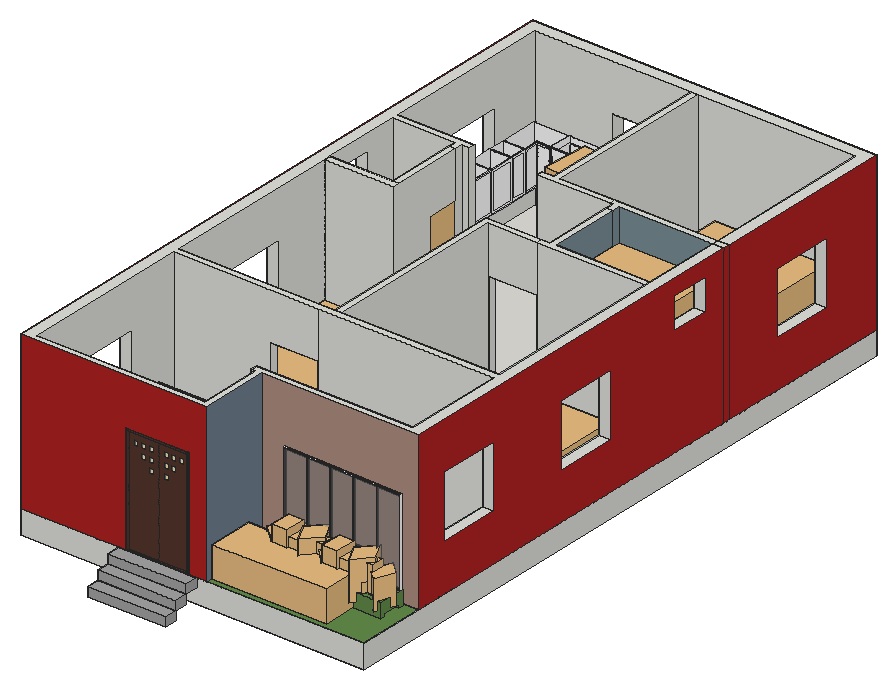
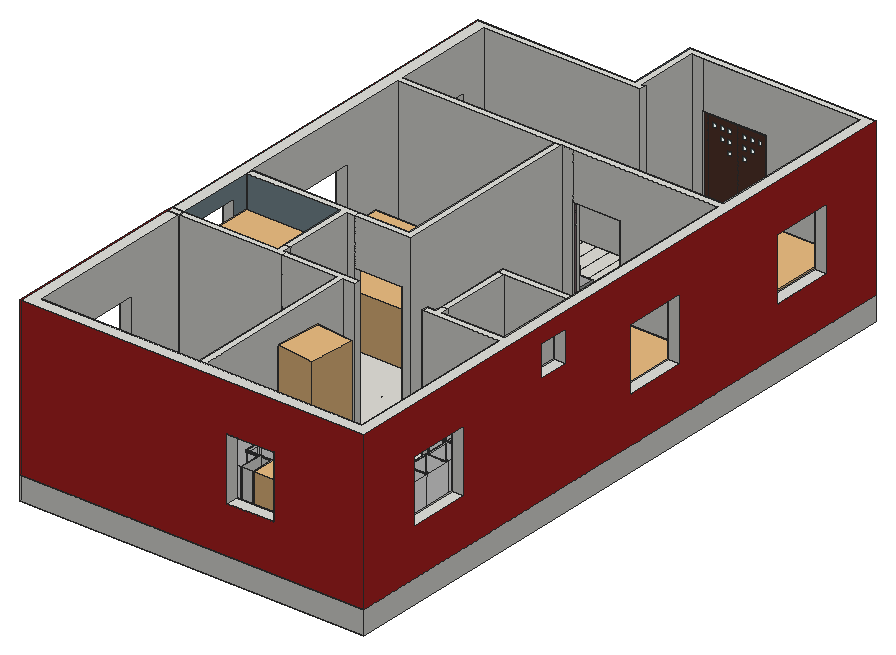
# SketchUp Ruby script. Lengths in inches.
U = 1.inch
M = Sketchup.active_model
def pt(a) = Geom::Point3d.new(a.map { |v| v * U })
def face(e, loops, mat)
  f = e.add_face(loops[0].map { |a| pt(a) })
  loops[1..].each { |l| e.add_face(l.map { |a| pt(a) }).erase! }
  f.material = f.back_material = mat if mat
  f
end
# faces: each face lists its corners as indices into pts; further lists are holes
def faces(e, pts, list, mat = nil) = list.each { |f| face(e, (f[0].is_a?(Array) ? f : [f]).map { |l| l.map { |i| pts[i] } }, mat) }
# xy, xz, yz: faces in a plane at the given z, y or x. An outline is a flat list of corners, or four numbers for a rectangle; further outlines are holes
def ring(l) = l.size == 4 ? [[l[0], l[1]], [l[2], l[1]], [l[2], l[3]], [l[0], l[3]]] : l.each_slice(2).to_a
def flat(e, list, mat, &to3) = list.each { |f| face(e, (f[0].is_a?(Array) ? f : [f]).map { |l| ring(l).map { |u, v| to3.(u, v) } }, mat) }
def xy(e, z, list, mat = nil) = flat(e, list, mat) { |x, y| [x, y, z] }
def xz(e, y, list, mat = nil) = flat(e, list, mat) { |x, z| [x, y, z] }
def yz(e, x, list, mat = nil) = flat(e, list, mat) { |y, z| [x, y, z] }
def lines(e, pts, list) = list.each { |a, b| e.add_line(pt(pts[a]), pt(pts[b])) }
# prism: a flat outline (further loops are holes) pulled along v
def prism(e, loops, v, mat = nil)
  f = face(e, loops, mat); d = Geom::Vector3d.new(v.map { |x| x * U })
  f.pushpull(f.normal.samedirection?(d) ? d.length : -d.length)
end
def box(e, o, s, mat = nil) = prism(e, [[o, [o[0] + s[0], o[1], o[2]], [o[0] + s[0], o[1] + s[1], o[2]], [o[0], o[1] + s[1], o[2]]]], [0, 0, s[2]], mat)
def at(x, y, z, deg = 0) = Geom::Transformation.translation(pt([x, y, z])) * Geom::Transformation.rotation(ORIGIN, Z_AXIS, deg.degrees)
def axes(o, x, y, z) = Geom::Transformation.new([*x, 0, *y, 0, *z, 0, *pt(o).to_a, 1])
def part(name) = M.definitions.add(name)
# library, detail: a bought-in or finely detailed component or shape, given as its bounding box
def library(name, o, s) = part(name).tap { |d| box(d.entities, o, s) }
def detail(e, o, s) = box(e.add_group.entities, o, s)
def put(e, d, t, mat = nil) = e.add_instance(d, t).tap { |i| i.material = mat if mat }
def group(e, t, mat = nil) = e.add_group.tap { |g| g.transformation = t; g.material = mat if mat }.entities
root = M.entities
M.materials.add("0128_White").color = [255, 255, 255]
M.materials.add("20200827_091549.jpgrr").color = [163, 138, 121]
M.materials.add("Material__1").color = [95, 70, 46]
M.materials.add("Steve_Hair1").color = [228, 228, 225]
M.materials.add("[0023_FireBrick]").color = [178, 34, 34]
M.materials.add("[0111_SlateGray]").color = [112, 128, 144]
M.materials.add("[Color M00]2").color = [255, 255, 255]
M.materials.add("[Color_H05]").color = [204, 255, 255]
M.materials["[Color_H05]"].alpha = 0.3
M.materials.add("[Marble Carrara Gold Floor Tile]").color = [225, 223, 217]
M.materials.add("[Pavers Modular Brick]").color = [175, 143, 129]
M.materials.add("[Square Glass Tile 01]").color = [123, 142, 151]
M.materials.add("[Stone Vein Gray]").color = [166, 165, 165]
M.materials.add("[Translucent Glass Gray]").color = [128, 128, 128]
M.materials["[Translucent Glass Gray]"].alpha = 0.29
M.materials.add("[Vegetation Grass Artificial]").color = [98, 140, 74]
M.materials.add("[Wood Veneer 01]").color = [120, 70, 37]
M.materials.add("[sketch-stone]").color = [126, 99, 107]
M.materials.add("big").color = [85, 54, 44]
M.materials.add("wood").color = [255, 255, 255]
c1 = part("Group\#7")
box(c1.entities,[0,0,0],[60,10,7])
c2 = library("The whole professional bed",[-16.91,-10.3,-0.31],[85.22,91.2,40.45])
c3 = library("36",[-44.7,-74.43,-0.38],[89.21,170.96,60.16])
c4 = library("Door C1",[0,0,0],[35.43,8.39,80.71])
c5 = part("main door")
xy(c5.entities,0,[[0,0,3.9375,70.87]],"big")
xy(c5.entities,0.35,[[0,1.38,1.97,35.43],[1.97,1.38,3.9375,35.43],[0,35.43,1.97,69.49],[1.97,35.43,3.9375,69.49]],"big")
xy(c5.entities,93.11,[[0,1.38,1.97,35.43],[1.97,1.38,3.9375,35.43],[0,35.43,1.97,69.49],[1.97,35.43,3.9375,69.49]],"big")
xy(c5.entities,94.49,[[0,0,3.9375,70.87]],"big")
xz(c5.entities,0,[[0,0,3.9375,94.49]],"big")
xz(c5.entities,1.38,[[0,0.35,1.97,93.11],[1.97,0.35,3.9375,93.11]],"big")
xz(c5.entities,69.49,[[0,0.35,1.97,93.11],[1.97,0.35,3.9375,93.11]],"big")
xz(c5.entities,70.87,[[0,0,3.9375,94.49]],"big")
yz(c5.entities,0,[[[0,0,70.87,94.49],[1.38,0.35,69.49,93.11]]],"big")
yz(c5.entities,1.97,[[41.69,64.73,45.9,68.94],[24.84,64.85,29.05,69.06],[41.69,73.35,45.9,77.5625],[50.23,73.35,54.45,77.5625],[16.0625,73.43,20.27,77.64],
  [24.84,73.43,29.05,77.64],[7.48,81.93,11.69,86.14],[16.0625,81.93,20.27,86.14],[24.84,81.93,29.05,86.14],[41.69,81.93,45.9,86.14],
  [50.23,81.93,54.45,86.14],[58.82,81.93,63.03,86.14]],"[Color_H05]")
yz(c5.entities,1.97,[[[1.38,0.35,35.43,93.11],[24.84,81.93,29.05,86.14],[16.0625,81.93,20.27,86.14],[7.48,81.93,11.69,86.14],[24.84,73.43,29.05,77.64],[16.0625,73.43,20.27,77.64],[24.84,64.85,29.05,69.06]],[[35.43,0.35,69.49,93.11],[41.69,81.93,45.9,86.14],[50.23,81.93,54.45,86.14],[58.82,81.93,63.03,86.14],[50.23,73.35,54.45,77.5625],[41.69,73.35,45.9,77.5625],[41.69,64.73,45.9,68.94]]],"big")
yz(c5.entities,3.9375,[[[0,0,70.87,94.49],[1.38,0.35,69.49,93.11]]],"big")
c6 = part("d1")
xy(c6.entities,0,[[0,0,18,1.6],[18,0,36,1.6]],"[sketch-stone]")
xy(c6.entities,72,[[0,0,18,1.6],[18,0,36,1.6]],"[sketch-stone]")
yz(c6.entities,0,[[0,0,1.6,72]],"[sketch-stone]")
yz(c6.entities,36,[[0,0,1.6,72]],"[sketch-stone]")
c7 = library("Dining table set",[-3.55,-0.1,0],[135.47,90.42,53.12])
c8 = part("Group\#5")
box(c8.entities,[0,0,0],[10.125,36,6])
c9 = library("Group\#61",[0,0,0],[50.37,77,85.15])
c10 = library("Group\#183",[-0.62,0,0],[57,79.03,20.625])
c11 = library("Areca palm plant",[0,0,0],[49.1,36.6,54.46])
c12 = part("W1")
xy(c12.entities,15,[[0,0,2,198]])
xy(c12.entities,102.0625,[[0,0,2,198]],"[Color M00]2")
xz(c12.entities,0,[[0,15,2,102.0625]],"[Color M00]2")
xz(c12.entities,198,[[0,15,2,102.0625]])
yz(c12.entities,0,[[0.84,16,39.43,101.0625],[40.28,16,78.87,101.0625],[79.71,16,118.3,101.0625],[119.14,16,157.73,101.0625],[158.58,16,197.16,101.0625]])
yz(c12.entities,0,[[[0,15,198,102.0625],[0.84,16,197.16,101.0625]],[39.43,16,40.28,101.0625],[78.87,16,79.71,101.0625],[118.3,16,119.14,101.0625],[157.73,16,158.58,101.0625]],"[Color M00]2")
yz(c12.entities,2,[[0.84,16,39.43,101.0625],[40.28,16,78.87,101.0625],[79.71,16,118.3,101.0625],[119.14,16,157.73,101.0625],[158.58,16,197.16,101.0625]])
yz(c12.entities,2,[[[0,15,198,102.0625],[0.84,16,197.16,101.0625]],[39.43,16,40.28,101.0625],[78.87,16,79.71,101.0625],[118.3,16,119.14,101.0625],[157.73,16,158.58,101.0625]],"[Color M00]2")
c13 = library("Group\#220",[-84.69,-90.07,-0.36],[176.51,175.13,171.4])
c14 = library("Group20\#1",[-20.81,-17.08,3.79],[39.86,39.43,37.51])
c15 = library("Group\#221",[-7.34,-1.2,0],[38.67,35.81,49.04])
c16 = library("Group38\#2",[14.01,28.44,-23.43],[18.58,18.32,38.89])
c17 = part("PLANTS")
put(c17.entities,c11,axes([38.49,169.84,6.02],[0.45017,-0.56191,0],[0.66137,0.52986,0],[0,0,0.72]))
put(c17.entities,c11,axes([38.49,68.02,6.02],[0.45017,-0.56191,0],[0.66137,0.52986,0],[0,0,0.72]))
put(c17.entities,c12,axes([76.68,11.43,-0.0625],[1,0,0],[0,1.18586,0],[0,0,1]),"[Translucent Glass Gray]")
put(c17.entities,c13,axes([59.61,184.54,5.99],[-0.04961,-0.08593,0],[0.08593,-0.04961,0],[0,0,0.10522]))
put(c17.entities,c13,axes([59.61,204.61,5.99],[-0.04961,-0.08593,0],[0.08593,-0.04961,0],[0,0,0.10522]))
put(c17.entities,c13,axes([59.61,157.29,5.99],[-0.04961,-0.08593,0],[0.08593,-0.04961,0],[0,0,0.10522]))
put(c17.entities,c14,axes([63.65,91.4,4.71],[0,0.85,0],[-0.85,0,0],[0,0,0.85]))
put(c17.entities,c15,axes([69.62,101.34,7.93],[0,0.79,0],[-0.79,0,0],[0,0,0.79]))
put(c17.entities,c16,axes([40.58,10.27,28.11],[0.8848,0,0],[0,0.94674,0],[0,0,0.85826]))
put(c17.entities,c13,axes([59.61,55.48,5.99],[-0.04961,-0.08593,0],[0.08593,-0.04961,0],[0,0,0.10522]))
put(c17.entities,c13,axes([59.61,82.73,5.99],[-0.04961,-0.08593,0],[0.08593,-0.04961,0],[0,0,0.10522]))
put(c17.entities,c13,axes([61.875,132.66,6.01],[-0.08133,-0.14087,0],[0.14087,-0.08133,0],[0,0,0.1725]))
put(c17.entities,c13,axes([59.61,102.79,5.99],[-0.04961,-0.08593,0],[0.08593,-0.04961,0],[0,0,0.10522]))
put(c17.entities,c13,axes([61.875,27.22,6.01],[-0.08133,-0.14087,0],[0.14087,-0.08133,0],[0,0,0.1725]))
put(c17.entities,c13,axes([61.875,234.47,6.01],[-0.08133,-0.14087,0],[0.14087,-0.08133,0],[0,0,0.1725]))
put(c17.entities,c15,axes([69.62,203.15,7.93],[0,0.79,0],[-0.79,0,0],[0,0,0.79]))
put(c17.entities,c14,axes([63.65,193.21,4.71],[0,0.85,0],[-0.85,0,0],[0,0,0.85]))
put(c17.entities,c16,axes([40.58,112.08,28.11],[0.8848,0,0],[0,0.94674,0],[0,0,0.85826]))
g1 = group(c17.entities,at(44.68,11.43,-0.0625))
xy(g1,0,[[0,0,6,234.8],[30,0,36,234.8]])
xy(g1,3,[[6,0,30,234.8]])
xy(g1,7,[[6,5,30,229.8]],"Material__1")
xy(g1,15,[[[0,0,36,234.8],[6,5,30,229.8]]])
xz(g1,0,[[0,0,6,0,6,3,30,3,30,0,36,0,36,15,0,15]])
xz(g1,5,[[6,7,30,15]])
xz(g1,229.8,[[6,7,30,15]])
xz(g1,234.8,[[0,0,0,15,36,15,36,0,30,0,30,3,6,3,6,0]])
yz(g1,0,[[0,0,234.8,15]])
yz(g1,6,[[0,0,234.8,3],[5,7,229.8,15]])
yz(g1,30,[[0,0,234.8,3],[5,7,229.8,15]])
yz(g1,36,[[0,0,234.8,15]])
c18 = library("Group\#182",[0,0,0],[82.79,96.12,21.4])
c19 = part("550 X 309 back")
box(c19.entities,[0,0.51,0],[12.17,0.12,34.25])
c20 = part("550 X 309 side")
prism(c20.entities,[[[0.63,0,34.25],[0.63,0,3.9375],[0.63,4.57,3.9375],[0.63,4.57,0],[0.63,21.54,0],[0.63,21.54,34.25]]],[-0.63,0,0])
c21 = part("550 X 309 cabinet door")
xy(c21.entities,1.63,[[-15.83,0,14.17,0.63]])
xy(c21.entities,13.17,[[-15.83,0,14.17,0.63]])
xz(c21.entities,0,[[-15.83,1.63,14.17,13.17]])
xz(c21.entities,0.63,[[[-15.83,1.63,14.17,13.17],[-14.65,2.8125,12.99,11.98]],[-14.65,2.8125,12.99,11.98]])
yz(c21.entities,-15.83,[[0,1.63,0.63,13.17]])
yz(c21.entities,14.17,[[0,1.63,0.63,13.17]])
c22 = part("550 X 309 top s")
box(c22.entities,[0,0,0],[10.91,0.63,0.63])
c23 = part("550 X 309 bottom")
box(c23.entities,[0,0,0],[10.91,21.54,0.63])
c24 = part("550 X 309 floor front")
box(c24.entities,[0,0,0],[12.17,0.63,3.9375])
c25 = part("550 X 600 side\#1")
prism(c25.entities,[[[0.63,0,34.25],[0.63,0,3.9375],[0.63,4.57,3.9375],[0.63,4.57,0],[0.63,21.54,0],[0.63,21.54,34.25]]],[-0.63,0,0])
c26 = part("550 X 600 side")
put(c26.entities,c25,at(0,0,0),"wood")
c27 = part("550 X600 mid shelf")
box(c27.entities,[0,0,0],[22.36,20.91,0.63])
c28 = part("550 X 600 back")
box(c28.entities,[0,0.51,0],[23.62,0.12,34.25])
c29 = part("550 X600 back")
g2 = group(c29.entities,at(0,0,0))
put(g2,c28,at(0,0,0),"wood")
c30 = part("550 X 600 floor front")
box(c30.entities,[0,0,0],[23.62,0.63,3.9375])
c31 = part("unit a1 support")
box(c31.entities,[0,0,0],[22.36,0.63,0.63])
c32 = part("550 X 600 top s")
put(c32.entities,c31,at(0,0,0),"wood")
c33 = part("550 X 600 bottom")
box(c33.entities,[0,0,0],[22.36,21.5,0.63],"0128_White")
c34 = part("550 X 600 cabint  door")
xy(c34.entities,0,[[-15.83,0,14.17,0.63]])
xy(c34.entities,22.99,[[-15.83,0,14.17,0.63]])
xz(c34.entities,0,[[-15.83,0,14.17,22.99]])
xz(c34.entities,0.63,[[[-15.83,0,14.17,22.99],[-14.65,1.18,12.99,21.8125]],[-14.65,1.18,12.99,21.8125]])
yz(c34.entities,-15.83,[[0,0,0.63,22.99]])
yz(c34.entities,14.17,[[0,0,0.63,22.99]])
c35 = part("cabiner 550 X 600")
put(c35.entities,c26,at(0,0,0))
put(c35.entities,c27,at(0.63,0.63,21.38),"wood")
put(c35.entities,c29,at(0,21.02,0))
put(c35.entities,c30,at(0,3.9375,0),"wood")
put(c35.entities,c32,at(0.63,0,33.62))
put(c35.entities,c33,at(0.63,0.04,3.9375),"wood")
put(c35.entities,c34,axes([23.31,0,18.11],[0,0,-1],[0,-1,0],[-1,0,0]),"wood")
put(c35.entities,c26,at(22.99,0,0))
c36 = library("Group\#96",[0,0,0],[23.62,24.72,34.25])
c37 = part("550 x 800 side\#1")
prism(c37.entities,[[[0,0,3.9375],[0,0,34.25],[0,21.54,34.25],[0,21.54,0],[0,4.57,0],[0,4.57,3.9375]]],[0.63,0,0])
c38 = part("550 x 800 bottom")
box(c38.entities,[0,-0.03,0],[30.24,21.53,0.63])
c39 = part("550 X 800 back")
box(c39.entities,[0,0.51,0],[31.5,0.12,34.25])
c40 = part("550 X 800 top  s")
xy(c40.entities,0,[[0,0,30.24,0.63]])
xy(c40.entities,0.63,[[0,0,30.24,0.63]])
xz(c40.entities,0,[[0,0,30.24,0.63]])
xz(c40.entities,0.63,[[0,0,30.24,0.63]],"20200827_091549.jpgrr")
yz(c40.entities,0,[[0,0,0.63,0.63]])
yz(c40.entities,30.24,[[0,0,0.63,0.63]])
c41 = part("550 X 800 floor front")
box(c41.entities,[0,0,0],[31.5,0.63,3.9375])
c42 = part("550 X 800 drawer back/front")
box(c42.entities,[0.04,20.39,0],[28.35,0.63,9.29],"wood")
c43 = part("550 X 800 drawer side")
box(c43.entities,[0,0,0],[0.63,21.02,9.92],"wood")
c44 = part("550 X 800 drawer bottom")
box(c44.entities,[0,0,0],[28.43,21.02,0.63],"wood")
c45 = part("550 X 600  drawer front")
xy(c45.entities,0,[[0,0,30.87,0.63]],"20200827_091549.jpgrr")
xy(c45.entities,14.84,[[0,0,30.87,0.63]],"20200827_091549.jpgrr")
xz(c45.entities,0,[[0,0,30.87,14.84]],"0128_White")
xz(c45.entities,0.63,[[0,0,30.87,14.84]],"0128_White")
yz(c45.entities,0,[[0,0,0.63,14.84]],"20200827_091549.jpgrr")
yz(c45.entities,30.87,[[0,0,0.63,14.84]],"20200827_091549.jpgrr")
c46 = part("500 X 800 drawer front face")
put(c46.entities,c45,at(0,0,0),"wood")
c47 = part("Group\#205")
put(c47.entities,c42,at(1.22,0,1.22),"wood")
put(c47.entities,c42,at(1.22,-20.39,1.22),"wood")
put(c47.entities,c43,at(29.61,0,0.59),"wood")
put(c47.entities,c43,at(0.63,0,0.59),"wood")
put(c47.entities,c44,at(1.22,0,0.63),"wood")
put(c47.entities,c46,at(0,21.02,-0.16),"0128_White")
c48 = part("550 x 500 back")
box(c48.entities,[-0.63,0.51,0],[19.69,0.12,34.25])
c49 = part("550 X 500 side")
prism(c49.entities,[[[0,0,3.9375],[0,0,34.25],[0,21.54,34.25],[0,21.54,0],[0,4.57,0],[0,4.57,3.9375]]],[0.63,0,0])
c50 = part("550 X 500 bottom")
box(c50.entities,[-0.63,0,0],[18.43,21.54,0.63])
c51 = part("550 X 500 cabinet door")
xy(c51.entities,4.57,[[-15.83,0,14.17,0.63]])
xy(c51.entities,23.62,[[-15.83,0,14.17,0.63]])
xz(c51.entities,0,[[-15.83,4.57,14.17,23.62]])
xz(c51.entities,0.63,[[[-15.83,4.57,14.17,23.62],[-14.65,5.75,12.99,22.44]],[-14.65,5.75,12.99,22.44]])
yz(c51.entities,-15.83,[[0,4.57,0.63,23.62]])
yz(c51.entities,14.17,[[0,4.57,0.63,23.62]])
c52 = part("550 X 500 top s")
box(c52.entities,[-0.63,0,0],[18.43,0.63,0.63])
c53 = part("550X 500 floor front")
box(c53.entities,[-0.63,0,0],[19.69,0.63,3.9375])
c54 = part("550 X 500 mid shelf")
box(c54.entities,[-0.63,0.31,0],[18.43,21.23,0.63])
c55 = part("corner cabinet back")
box(c55.entities,[0,0.63,0],[0.12,35.31,34.25])
c56 = part("corner cabinet floor front")
box(c56.entities,[0,0.63,0],[0.63,17.72,3.9375])
c57 = part("corner cabinet top s1")
box(c57.entities,[0,0.63,0],[0.63,13.15,0.63])
c58 = part("corner cabinet top s2")
box(c58.entities,[0,0,0],[0.63,13.78,0.63])
c59 = part("corner cabinet side")
prism(c59.entities,[[[0,0,3.9375],[0,0,34.25],[0,21.54,34.25],[0,21.54,0],[0,4.57,0],[0,4.57,3.9375]]],[0.63,0,0])
c60 = part("corner cabiner back 2")
box(c60.entities,[-0.63,0.51,0],[35.43,0.12,34.25])
c61 = part("corner cabinet bottom")
prism(c61.entities,[[[-0.51,35.31,-0.63],[34.17,35.31,-0.63],[34.17,13.78,-0.63],[21.02,13.78,-0.63],[21.02,0.63,-0.63],[-0.51,0.63,-0.63]]],[0,0,0.63])
c62 = part("corner cabinet door 2")
xy(c62.entities,0.31,[[-15.83,0,14.17,0.63]])
xy(c62.entities,12.875,[[-15.83,0,14.17,0.63]])
xz(c62.entities,0,[[-15.83,0.31,14.17,12.875]])
xz(c62.entities,0.63,[[[-15.83,0.31,14.17,12.875],[-14.65,1.5,12.99,11.98]],[-14.65,1.5,12.99,11.98]])
yz(c62.entities,-15.83,[[0,0.31,0.63,12.875]])
yz(c62.entities,14.17,[[0,0.31,0.63,12.875]])
c63 = part("corner cabinet door 1")
xy(c63.entities,-0.18,[[-15.83,0,14.17,0.63]])
xy(c63.entities,13.17,[[-15.83,0,14.17,0.63]])
xz(c63.entities,0,[[-15.83,-0.18,14.17,13.17]])
xz(c63.entities,0.63,[[[-15.83,-0.18,14.17,13.17],[-14.65,1,12.99,11.98]],[-14.65,1,12.99,11.98]])
yz(c63.entities,-15.83,[[0,-0.18,0.63,13.17]])
yz(c63.entities,14.17,[[0,-0.18,0.63,13.17]])
c64 = part("corner cabinet")
put(c64.entities,c55,at(0,0,0),"wood")
put(c64.entities,c56,at(17.09,0,0),"wood")
put(c64.entities,c57,at(21.02,0.63,33.62),"wood")
put(c64.entities,c58,at(34.8,14.41,33.62,90),"wood")
put(c64.entities,c59,at(34.8,14.41,0),"wood")
put(c64.entities,c60,at(0.63,35.43,0),"wood")
put(c64.entities,c56,at(17.09,18.98,0,-90),"wood")
put(c64.entities,c59,at(21.65,0.63,0,90),"wood")
put(c64.entities,c61,at(0.63,0.63,4.57),"wood")
put(c64.entities,c62,axes([35.45,14.41,18.11],[0,0,-1],[0,-1,0],[-1,0,0]),"wood")
put(c64.entities,c63,axes([21.65,14.11,18.11],[0,0,-1],[1,0,0],[0,-1,0]),"wood")
c65 = library("High tech Frige",[11.53,-10.51,0],[42.41,37.43,78.625])
c66 = part("550 X 450 drawer back/ front")
box(c66.entities,[0,0,-0.51],[14.61,0.63,5.43],"wood")
c67 = part("550 X 450 drawer side")
box(c67.entities,[0,0,0.12],[0.63,20.39,5.43],"0128_White")
c68 = part("550 X 450 drawer bottom")
xy(c68.entities,0,[[-0.63,0,15.24,20.39]],"0128_White")
xy(c68.entities,0.12,[[-0.63,0,15.24,20.39]],"0128_White")
xz(c68.entities,0,[[-0.63,0,15.24,0.12]],"20200827_091549.jpgrr")
xz(c68.entities,20.39,[[-0.63,0,15.24,0.12]],"20200827_091549.jpgrr")
yz(c68.entities,-0.63,[[0,0,20.39,0.12]],"20200827_091549.jpgrr")
yz(c68.entities,15.24,[[0,0,20.39,0.12]],"20200827_091549.jpgrr")
c69 = part("550 X 450 drawer front face")
xy(c69.entities,0,[[0,0,17.09,0.63]])
xy(c69.entities,7.26,[[0,0,17.09,0.63]])
xz(c69.entities,0,[[[0,0,17.09,7.26],[1.18,1.18,15.91,6.08]],[1.18,1.18,15.91,6.08]])
xz(c69.entities,0.63,[[0,0,17.09,7.26]])
yz(c69.entities,0,[[0,0,0.63,7.26]])
yz(c69.entities,17.09,[[0,0,0.63,7.26]])
c70 = part("Group\#72")
put(c70.entities,c66,at(1.08,20.39,1.26),"wood")
put(c70.entities,c66,at(1.08,0.63,1.26),"wood")
put(c70.entities,c67,at(15.6875,0.63,0.63),"wood")
put(c70.entities,c67,at(0.45,0.63,0.63),"wood")
put(c70.entities,c68,at(1.08,0.63,0.63),"wood")
put(c70.entities,c69,at(-0.31,0,0),"wood")
c71 = part("550 X 450 bottom")
box(c71.entities,[13.78,0,0],[16.46,21.02,0.63])
c72 = part("550 X 450 side")
prism(c72.entities,[[[0,21.02,34.25],[0,21.02,3.9375],[0,16.46,3.9375],[0,16.46,0],[0,-0.51,0],[0,-0.51,34.25]]],[0.63,0,0])
c73 = part("550 X 450 floor front")
box(c73.entities,[0,0,0],[17.72,0.63,3.9375])
c74 = part("550 X 450 back")
box(c74.entities,[0,0,0],[17.72,0.12,34.25])
c75 = part("550 X 450 top s")
box(c75.entities,[0,0,0],[16.46,0.63,0.63])
c76 = part("550 X 450 draer bottom")
box(c76.entities,[13.9375,0,0],[16.14,20.71,0.63])
c77 = part("550 X 450 cabinet door")
xy(c77.entities,0,[[0,0,17.09,0.63]])
xy(c77.entities,30,[[0,0,17.09,0.63]])
xz(c77.entities,0,[[[0,0,17.09,30],[1.18,1.18,15.91,28.82]],[1.18,1.18,15.91,28.82]],"0128_White")
xz(c77.entities,0.63,[[0,0,17.09,30]],"0128_White")
yz(c77.entities,0,[[0,0,0.63,30]])
yz(c77.entities,17.09,[[0,0,0.63,30]])
c78 = part("Component\#15")
box(c78.entities,[0,0.63,0],[0.63,20.08,17.72])
c79 = part("550 X 450 draer front.")
box(c79.entities,[0,0,0],[16.14,0.63,25.59])
c80 = part("550 X 400 side")
prism(c80.entities,[[[0.63,0,34.25],[0.63,0,3.9375],[0.63,4.57,3.9375],[0.63,4.57,0],[0.63,21.54,0],[0.63,21.54,34.25]]],[-0.63,0,0])
c81 = part("550 X 400 back")
box(c81.entities,[0,0.51,0],[15.75,0.12,34.25])
c82 = part("550 X 400 bottom")
box(c82.entities,[0,0,0],[14.49,21.54,0.63])
c83 = part("550 X 400 top s")
box(c83.entities,[0,0,0],[14.49,0.63,0.63])
c84 = part("550 X 400  cabinet door")
xy(c84.entities,-1.65,[[-15.83,0,14.17,0.63]])
xy(c84.entities,13.46,[[-15.83,0,14.17,0.63]])
xz(c84.entities,0,[[-15.83,-1.65,14.17,13.46]])
xz(c84.entities,0.63,[[[-15.83,-1.65,14.17,13.46],[-14.65,-0.47,12.99,12.28]],[-14.65,-0.47,12.99,12.28]])
yz(c84.entities,-15.83,[[0,-1.65,0.63,13.46]])
yz(c84.entities,14.17,[[0,-1.65,0.63,13.46]])
c85 = part("550 X 400 front floor")
box(c85.entities,[0,0,0],[15.75,0.63,3.9375])
c86 = part("550 x 400 mid shelf\#1")
box(c86.entities,[0,0.31,0],[14.49,21.23,0.63])
xy(root,-18,[[0,30,264,522]])
xy(root,0,[[0,30,143,30,143,83,264,83,264,522,0,522]],"[Marble Carrara Gold Floor Tile]")
xy(root,0,[[143,30,264,83]],"[Vegetation Grass Artificial]")
xz(root,30,[[0,-18,264,0]])
xz(root,522,[[0,-18,264,0]])
yz(root,0,[[30,-18,522,0]])
yz(root,264,[[30,-18,522,0]])
put(root,c1,at(75.51,0,-21),"[Stone Vein Gray]")
put(root,c1,at(75.51,10,-14),"[Stone Vein Gray]")
put(root,c1,at(75.51,20,-7),"[Stone Vein Gray]")
put(root,c2,at(167.02,428.46,0))
put(root,c2,at(174.1,260.43,0.31,-90))
put(root,c3,axes([181.73,52.19,0.15],[0,-0.39161,0],[0.51415,0,0],[0,0,0.39161]))
put(root,c4,axes([178.5,370,0],[0,-0.67733,0],[0.53605,0,0],[0,0,1.04078]))
put(root,c4,axes([57.0625,370,0],[0,-0.67733,0],[0.58819,0,0],[0,0,1.04078]))
put(root,c5,axes([81,33.9375,0],[0,-1,0],[0.68,0,0],[0,0,0.889]))
put(root,c6,axes([140,376,0],[1,0,0],[0,3.125,0],[0,0,1.16667]))
put(root,c6,axes([136,312.83,0],[1,0,0],[0,1,0],[0,0,1.16667]))
put(root,c6,axes([84,168.125,0],[1,0,0],[0,1,0],[0,0,1.16667]))
put(root,c7,axes([10.5625,271.26,0],[0.44,0,0],[0,0.44,0],[0,0,0.44]))
g3 = group(root,at(0,30,0))
xy(g3,0,[[0,0,0,492,264,492,264,351,255,351,255,483,9,483,9,351,68,351,68,346,62,346,62,340,57,340,57,346,9,346,9,141,84,141,84,136,9,136,9,5,81,5,81,0],[129,0,129,5,138,5,138,53,135,53,135,58,255,58,255,136,120,136,120,141,255,141,255,346,264,346,264,53,143,53,143,0],[129,141,129,286,136,286,136,281,134,281,134,141],[9,281,62,286],[172,281,172,286,178,286,178,316,183,316,183,286,255,286,255,281],
  [57,286,62,316],[178,340,178,346,176,346,176,351,255,351,255,346,183,346,183,340],[120,346,120,351,129,351,129,483,134,483,134,351,140,351,140,346]])
xy(g3,2.8125,[[183,286,255,346]],"[Square Glass Tile 01]")
xy(g3,36,[[0,48,9,96],[255,77,264,125],[0,189,9,237],[255,189,264,237],[0,396,9,444],
  [255,396,264,444],[69,483,105,492]])
xy(g3,84,[[81,0,129,5],[0,48,9,96],[255,77,264,125],[84,136,120,141],[0,189,9,237],
  [255,189,264,237],[136,281,172,286],[0,298,9,322],[255,298,264,328],[57,316,62,340],
  [178,316,183,340],[140,346,176,351],[0,396,9,444],[255,396,264,444],[69,483,105,492]])
xy(g3,108,[[0,298,9,322],[255,298,264,328]])
xy(g3,120,[[0,0,143,0,143,53,264,53,264,346,255,346,255,141,120,141,120,136,255,136,255,58,135,58,135,53,138,53,138,5,9,5,9,136,120,136,120,141,9,141,9,346,57,346,57,340,62,340,62,346,68,346,68,351,9,351,9,483,255,483,255,351,264,351,264,492,0,492],[129,141,134,141,134,281,172,281,172,286,129,286],[9,281,62,286],[172,281,255,281,255,286,183,286,183,340,178,340,178,286,172,286],[57,286,62,340],
  [178,340,183,340,183,346,255,346,255,351,176,351,176,346,178,346],[120,346,176,346,176,351,134,351,134,483,129,483,129,351,120,351],[255,346,264,351]])
xz(g3,0,[[0,0,81,0,81,84,129,84,129,0,143,0,143,120,0,120]],"[0023_FireBrick]")
xz(g3,5,[[9,0,9,120,129,120,129,84,81,84,81,0],[129,0,138,120]])
xz(g3,48,[[0,36,9,84]])
xz(g3,53,[[135,0,138,120]])
xz(g3,53,[[143,0,264,120]],"[Pavers Modular Brick]")
xz(g3,58,[[135,0,255,120]])
xz(g3,77,[[255,36,264,84]])
xz(g3,96,[[0,36,9,84]])
xz(g3,125,[[255,36,264,84]])
xz(g3,136,[[9,0,84,0,84,84,120,84,120,120,9,120],[120,0,255,120]])
xz(g3,141,[[9,0,9,120,120,120,120,84,84,84,84,0],[120,0,129,120],[129,0,134,120],[134,0,255,120]])
xz(g3,189,[[0,36,9,84],[255,36,264,84]])
xz(g3,237,[[0,36,9,84],[255,36,264,84]])
xz(g3,281,[[9,0,62,120],[134,0,136,0,136,84,172,84,172,120,134,120],[172,0,255,120]])
xz(g3,286,[[9,0,57,120],[129,0,129,120,172,120,172,84,136,84,136,0],[172,0,178,120],[183,0,255,2.8125]])
xz(g3,286,[[183,2.8125,255,120]],"[Square Glass Tile 01]")
xz(g3,298,[[0,84,9,108],[255,84,264,108]])
xz(g3,316,[[57,0,62,84],[178,0,183,84]])
xz(g3,322,[[0,84,9,108]])
xz(g3,328,[[255,84,264,108]])
xz(g3,340,[[57,0,62,84],[178,0,183,84]])
xz(g3,346,[[9,0,57,120],[62,0,68,120],[120,0,140,0,140,84,176,84,176,120,120,120],[176,0,178,120],[183,0,255,2.8125],
  [255,0,264,120]])
xz(g3,346,[[183,2.8125,255,120]],"[Square Glass Tile 01]")
xz(g3,351,[[9,0,68,120],[120,0,129,120],[134,0,134,120,176,120,176,84,140,84,140,0],[176,0,255,120],[255,0,264,120]])
xz(g3,396,[[0,36,9,84],[255,36,264,84]])
xz(g3,444,[[0,36,9,84],[255,36,264,84]])
xz(g3,483,[[[9,0,129,120],[69,36,105,84]],[129,0,134,120],[134,0,255,120]])
xz(g3,492,[[[0,0,264,120],[69,36,105,84]]],"[0023_FireBrick]")
yz(g3,0,[[[0,0,492,120],[48,36,96,84],[189,36,237,84],[396,36,444,84],[298,84,322,108]]],"[0023_FireBrick]")
yz(g3,9,[[[5,0,136,120],[48,36,96,84]],[[141,0,281,120],[189,36,237,84]],[281,0,286,120],[[286,0,346,120],[298,84,322,108]],[[351,0,483,120],[396,36,444,84]]])
yz(g3,57,[[286,0,286,120,340,120,340,84,316,84,316,0],[340,0,346,120]])
yz(g3,62,[[281,0,316,0,316,84,340,84,340,120,281,120],[340,0,346,120]])
yz(g3,68,[[346,0,351,120]])
yz(g3,69,[[483,36,492,84]])
yz(g3,81,[[0,0,5,84]])
yz(g3,84,[[136,0,141,84]])
yz(g3,105,[[483,36,492,84]])
yz(g3,120,[[136,0,141,84],[346,0,351,120]])
yz(g3,129,[[0,0,5,84],[141,0,286,120],[351,0,483,120]])
yz(g3,134,[[141,0,281,120],[351,0,483,120]])
yz(g3,135,[[53,0,58,120]])
yz(g3,136,[[281,0,286,84]])
yz(g3,138,[[5,0,53,120]])
yz(g3,140,[[346,0,351,84]])
yz(g3,143,[[0,0,53,120]],"[0111_SlateGray]")
yz(g3,172,[[281,0,286,84]])
yz(g3,176,[[346,0,351,84]])
yz(g3,178,[[286,0,286,120,340,120,340,84,316,84,316,0],[340,0,346,120]])
yz(g3,183,[[286,0,316,2.8125],[340,0,346,2.8125]])
yz(g3,183,[[286,2.8125,316,2.8125,316,84,340,84,340,120,286,120],[340,2.8125,346,120]],"[Square Glass Tile 01]")
yz(g3,255,[[[58,0,136,120],[77,36,125,84]],[[141,0,281,120],[189,36,237,84]],[281,0,286,120],[286,0,346,2.8125],[346,0,351,120],
  [[351,0,483,120],[396,36,444,84]]])
yz(g3,255,[[[286,2.8125,346,120],[298,84,328,108]]],"[Square Glass Tile 01]")
yz(g3,264,[[[53,0,346,120],[189,36,237,84],[77,36,125,84],[298,84,328,108]],[346,0,351,120],[[351,0,492,120],[396,36,444,84]]],"[0023_FireBrick]")
p = [[264,0,0],[143,0,0],[264,53,0]]
lines(g3,p,[[0,1],[2,0]])
g4 = group(root,at(138,88,0))
p = [[70.875,42,0],[70.875,78,0],[60.75,42,0],[0,36,0],[10.125,36,0],[70.875,0,0],
  [70.875,36,0],[81,42,0],[81,78,0],[81,36,0],[50.625,42,0],[50.625,78,0],
  [30.375,42,0],[30.375,78,0],[20.25,42,0],[40.5,42,0],[81,0,0],[10.125,42,0],
  [60.75,78,0],[20.25,78,0],[10.125,78,0],[0,42,0],[40.5,78,0],[0,78,0],
  [10.125,0,0],[30.375,0,0],[30.375,36,0],[20.25,36,0],[40.5,0,0],[40.5,36,0],
  [0,0,0],[60.75,36,0],[50.625,0,0],[50.625,36,0],[60.75,0,0],[20.25,0,0]]
lines(g4,p,[[0,1],[0,2],[3,4],[5,6],[7,8],[9,7],[10,11],[12,13],[2,10],[12,14],[15,12],[16,9],
  [10,15],[14,17],[6,9],[2,18],[14,19],[17,20],[17,21],[15,22],[21,23],[24,4],[25,26],[4,27],
  [28,29],[26,29],[30,3],[7,0],[31,6],[21,3],[32,33],[34,31],[33,31],[29,33],[35,27],[27,26]])
put(root,c8,at(138,130,0),"[Stone Vein Gray]")
put(root,c9,axes([183,376,0],[0,-1.19125,0],[0.93506,0,0],[0,0,1.1214]))
put(root,c10,at(13.58,179.46,0))
put(root,c17,axes([257.04,33.64,0.05],[0.01501,0.5731,0],[-0.38987,0.01021,0],[0,0,0.76112]),"[Vegetation Grass Artificial]")
put(root,c8,at(148.125,130,6),"[Stone Vein Gray]")
put(root,c8,at(158.25,130,12),"[Stone Vein Gray]")
put(root,c18,at(9,55.4375,15.83))
put(root,c8,at(168.375,130,18),"[Stone Vein Gray]")
g5 = group(root,at(92.85,493.95,23.47),"Steve_Hair1")
put(g5,c19,axes([0,17.48,0],[0.75918,0,0],[0,0.8316,0],[0,0,1]))
put(g5,c20,axes([8.76,0,0],[0.75918,0,0],[0,0.8316,0],[0,0,1]))
put(g5,c20,axes([0,0,0],[0.75918,0,0],[0,0.8316,0],[0,0,1]))
put(g5,c21,axes([10.23,0,18.11],[0,0,-1],[0,-0.8316,0],[-0.75918,0,0]))
put(g5,c22,axes([0.48,0,33.62],[0.75918,0,0],[0,0.8316,0],[0,0,1]))
put(g5,c23,axes([0.48,0,3.9375],[0.75918,0,0],[0,0.8316,0],[0,0,1]))
put(g5,c24,axes([0,3.27,0],[0.75918,0,0],[0,0.8316,0],[0,0,1]))
put(root,c35,axes([112.55,482.49,23.47],[0,-0.8316,0],[0.75918,0,0],[0,0,1]),"Steve_Hair1")
put(root,c36,axes([74.92,491.4,23.47],[0.75918,0,0],[0,0.8316,0],[0,0,1]),"Steve_Hair1")
g6 = group(root,at(36.0625,493.4,23.47),"Steve_Hair1")
g7 = group(g6,at(0,0.55,0))
put(g7,c37,axes([0,0,0],[0.75918,0,0],[0,0.8316,0],[0,0,1]),"wood")
put(g7,c37,axes([23.43,0,0],[0.75918,0,0],[0,0.8316,0],[0,0,1]),"wood")
put(g7,c38,axes([0.48,0,3.9375],[0.75918,0,0],[0,0.8316,0],[0,0,1]),"wood")
put(g7,c39,axes([0,17.48,0],[0.75918,0,0],[0,0.8316,0],[0,0,1]),"wood")
put(g7,c40,axes([0.48,0,33.62],[0.75918,0,0],[0,0.8316,0],[0,0,1]),"wood")
put(g7,c41,axes([0,3.3,0],[0.75918,0,0],[0,0.8316,0],[0,0,1]),"wood")
put(g6,c47,axes([23.73,18.03,4.09],[-0.75918,0,0],[0,-0.8316,0],[0,0,1]),"20200827_091549.jpgrr")
put(g6,c47,axes([23.73,18.03,19.25],[-0.75918,0,0],[0,-0.8316,0],[0,0,1]),"20200827_091549.jpgrr")
g8 = group(root,at(60.45,493.95,23.47),"Steve_Hair1")
put(g8,c48,axes([0,17.48,0],[0.75918,0,0],[0,0.8316,0],[0,0,1]),"wood")
put(g8,c49,axes([-0.48,0,0],[0.75918,0,0],[0,0.8316,0],[0,0,1]),"wood")
put(g8,c49,axes([13.99,0,0],[0.75918,0,0],[0,0.8316,0],[0,0,1]),"wood")
put(g8,c50,axes([0.48,0,3.9375],[0.75918,0,0],[0,0.8316,0],[0,0,1]),"wood")
put(g8,c51,axes([17.69,0,18.11],[0,0,-1],[0,-0.8316,0],[-0.75918,0,0]),"wood")
put(g8,c52,axes([0.48,0,33.62],[0.75918,0,0],[0,0.8316,0],[0,0,1]),"wood")
put(g8,c53,axes([0,3.27,0],[0.75918,0,0],[0,0.8316,0],[0,0,1]),"wood")
put(g8,c54,axes([0.48,0,18.46],[0.75918,0,0],[0,0.8316,0],[0,0,1]),"wood")
put(root,c64,axes([9.16,481.97,23.47],[0.75918,0,0],[0,0.8316,0],[0,0,1]),"Steve_Hair1")
put(root,c35,axes([25.61,430.11,23.48],[0,0.8316,0],[-0.75918,0,0],[0,0,1]),"Steve_Hair1")
put(root,c35,axes([25.61,449.75,23.48],[0,0.8316,0],[-0.75918,0,0],[0,0,1]),"Steve_Hair1")
put(root,c64,axes([36.55,381,23.48],[0,0.8316,0],[-0.75918,0,0],[0,0,1]),"Steve_Hair1")
put(root,c35,axes([25.61,410.47,23.48],[0,0.8316,0],[-0.75918,0,0],[0,0,1]),"Steve_Hair1")
put(root,c65,axes([109.35,455.28,23.48],[-0.06353,-0.82868,0],[0.75652,-0.06959,0],[0,0,1]),"Steve_Hair1")
put(root,c64,axes([101.61,511.96,23.48],[0,-0.8316,0],[0.75918,0,0],[0,0,1]),"[Wood Veneer 01]")
g9 = group(root,at(128.99,448.12,23.48),"Steve_Hair1")
g10 = group(g9,at(-0.96,0.26,3.9375))
put(g10,c70,axes([-15.96,13.95,7.58],[0,-0.8316,0],[0.75918,0,0],[0,0,1]))
put(g10,c70,axes([-15.96,13.95,22.74],[0,-0.8316,0],[0.75918,0,0],[0,0,1]))
put(g10,c70,axes([-15.96,13.95,15.16],[0,-0.8316,0],[0.75918,0,0],[0,0,1]))
put(g10,c70,axes([-15.96,13.95,0],[0,-0.8316,0],[0.75918,0,0],[0,0,1]))
g11 = group(g9,at(0,0,0))
put(g11,c71,axes([-0.48,-10.94,3.9375],[0,0.8316,0],[-0.75918,0,0],[0,0,1]))
put(g11,c72,axes([-0.48,0,0],[0,0.8316,0],[-0.75918,0,0],[0,0,1]))
put(g11,c72,axes([-0.48,14.21,0],[0,0.8316,0],[-0.75918,0,0],[0,0,1]))
put(g11,c73,axes([-12.97,0,0],[0,0.8316,0],[-0.75918,0,0],[0,0,1]))
put(g11,c74,axes([0,0,0],[0,0.8316,0],[-0.75918,0,0],[0,0,1]))
put(g11,c75,axes([-15.96,0.52,33.62],[0,0.8316,0],[-0.75918,0,0],[0,0,1]))
g12 = group(root,at(36.08,399.53,23.48),"Steve_Hair1")
g13 = group(g12,at(-10.46,-18.01,0))
g14 = group(g13,at(10.46,-0.52,0))
put(g14,c71,axes([-9.98,0.52,3.9375],[0.75918,0,0],[0,0.8316,0],[0,0,1]),"wood")
put(g14,c72,axes([0,0.52,0],[0.75918,0,0],[0,0.8316,0],[0,0,1]),"wood")
put(g14,c72,axes([12.97,0.52,0],[0.75918,0,0],[0,0.8316,0],[0,0,1]),"wood")
put(g14,c73,axes([0,14.21,0],[0.75918,0,0],[0,0.8316,0],[0,0,1]),"wood")
put(g14,c74,axes([0,0,0],[0.75918,0,0],[0,0.8316,0],[0,0,1]),"wood")
put(g14,c75,axes([0.48,17.48,33.62],[0.75918,0,0],[0,0.8316,0],[0,0,1]),"wood")
g15 = group(g13,at(23.67,18.01,3.9375))
put(g15,c76,axes([10.22,-0.52,0.94],[-0.75918,0,0],[0,-0.8316,0],[0,0,1]),"wood")
put(g15,c77,axes([0,0,0],[-0.75918,0,0],[0,-0.8316,0],[0,0,1]),"wood")
put(g15,c78,axes([-0.36,-0.52,1.57],[-0.75918,0,0],[0,-0.8316,0],[0,0,1]),"wood")
put(g15,c78,axes([-12.13,-0.52,1.57],[-0.75918,0,0],[0,-0.8316,0],[0,0,1]),"wood")
put(g15,c79,axes([-0.36,-0.52,1.57],[-0.75918,0,0],[0,-0.8316,0],[0,0,1]),"wood")
g16 = group(root,at(25.61,469.4,23.48),"Steve_Hair1")
put(g16,c80,axes([0,0,0],[0,0.8316,0],[-0.75918,0,0],[0,0,1]),"wood")
put(g16,c80,axes([0,12.57,0],[0,0.8316,0],[-0.75918,0,0],[0,0,1]),"wood")
put(g16,c81,axes([-15.96,0,0],[0,0.8316,0],[-0.75918,0,0],[0,0,1]),"wood")
put(g16,c82,axes([0,0.52,3.9375],[0,0.8316,0],[-0.75918,0,0],[0,0,1]),"wood")
put(g16,c83,axes([0,0.52,33.62],[0,0.8316,0],[-0.75918,0,0],[0,0,1]),"wood")
put(g16,c84,axes([0,11.46,18.11],[0,0,-1],[0.75918,0,0],[0,-0.8316,0]),"wood")
put(g16,c85,axes([-2.99,0,0],[0,0.8316,0],[-0.75918,0,0],[0,0,1]),"wood")
put(g16,c86,axes([0,0.52,14.12],[0,0.8316,0],[-0.75918,0,0],[0,0,1]),"wood")
put(g16,c86,axes([0,0.52,24.63],[0,0.8316,0],[-0.75918,0,0],[0,0,1]),"wood")
